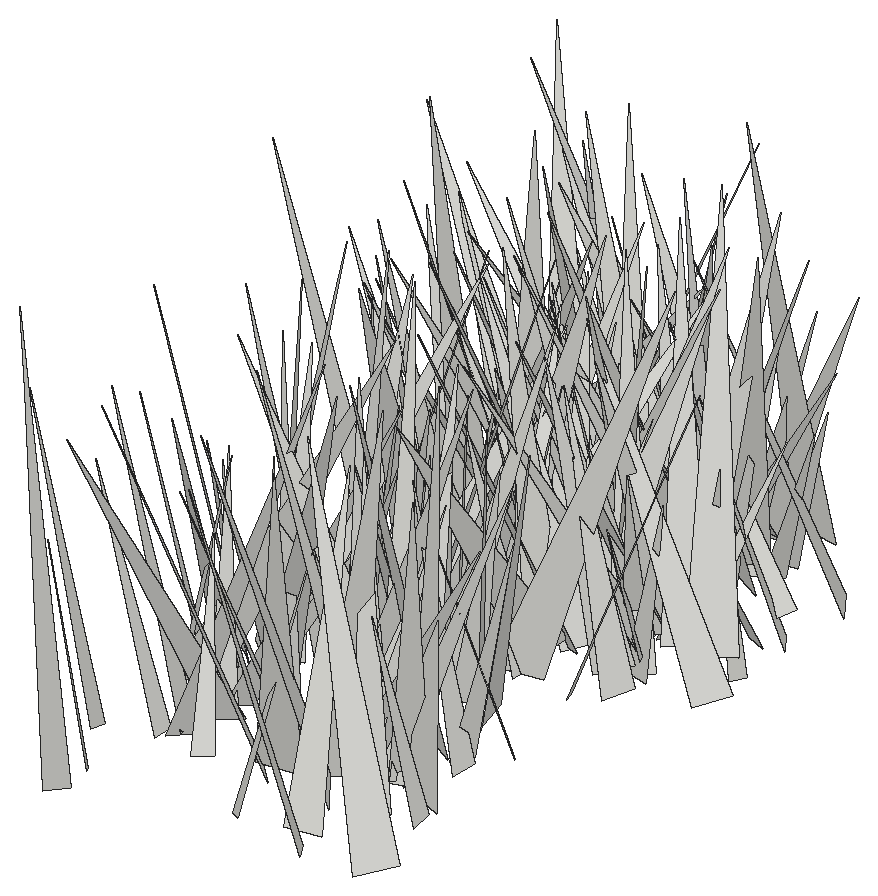
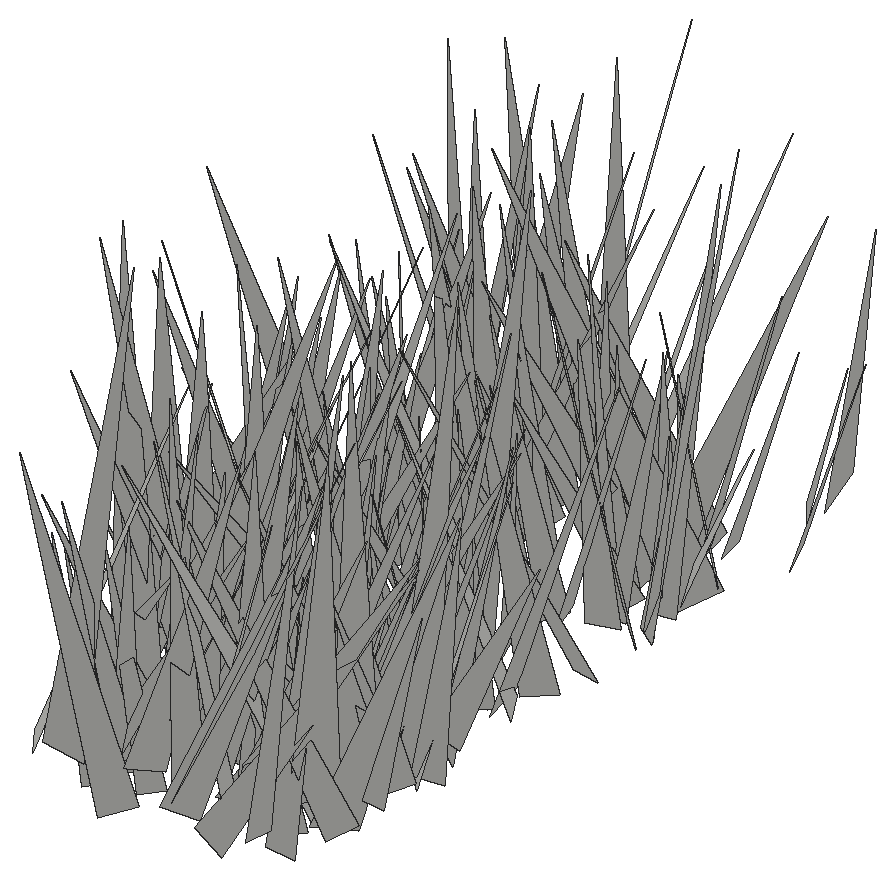
# SketchUp Ruby script. Lengths in inches.
U = 1.inch
M = Sketchup.active_model
def pt(a) = Geom::Point3d.new(a.map { |v| v * U })
def face(e, loops, mat)
  f = e.add_face(loops[0].map { |a| pt(a) })
  loops[1..].each { |l| e.add_face(l.map { |a| pt(a) }).erase! }
  f.material = f.back_material = mat if mat
  f
end
# faces: each face lists its corners as indices into pts; further lists are holes
def faces(e, pts, list, mat = nil) = list.each { |f| face(e, (f[0].is_a?(Array) ? f : [f]).map { |l| l.map { |i| pts[i] } }, mat) }
# xy, xz, yz: faces in a plane at the given z, y or x. An outline is a flat list of corners, or four numbers for a rectangle; further outlines are holes
def ring(l) = l.size == 4 ? [[l[0], l[1]], [l[2], l[1]], [l[2], l[3]], [l[0], l[3]]] : l.each_slice(2).to_a
def flat(e, list, mat, &to3) = list.each { |f| face(e, (f[0].is_a?(Array) ? f : [f]).map { |l| ring(l).map { |u, v| to3.(u, v) } }, mat) }
def xy(e, z, list, mat = nil) = flat(e, list, mat) { |x, y| [x, y, z] }
def xz(e, y, list, mat = nil) = flat(e, list, mat) { |x, z| [x, y, z] }
def yz(e, x, list, mat = nil) = flat(e, list, mat) { |y, z| [x, y, z] }
def lines(e, pts, list) = list.each { |a, b| e.add_line(pt(pts[a]), pt(pts[b])) }
# prism: a flat outline (further loops are holes) pulled along v
def prism(e, loops, v, mat = nil)
  f = face(e, loops, mat); d = Geom::Vector3d.new(v.map { |x| x * U })
  f.pushpull(f.normal.samedirection?(d) ? d.length : -d.length)
end
def box(e, o, s, mat = nil) = prism(e, [[o, [o[0] + s[0], o[1], o[2]], [o[0] + s[0], o[1] + s[1], o[2]], [o[0], o[1] + s[1], o[2]]]], [0, 0, s[2]], mat)
def at(x, y, z, deg = 0) = Geom::Transformation.translation(pt([x, y, z])) * Geom::Transformation.rotation(ORIGIN, Z_AXIS, deg.degrees)
def axes(o, x, y, z) = Geom::Transformation.new([*x, 0, *y, 0, *z, 0, *pt(o).to_a, 1])
def part(name) = M.definitions.add(name)
# library, detail: a bought-in or finely detailed component or shape, given as its bounding box
def library(name, o, s) = part(name).tap { |d| box(d.entities, o, s) }
def detail(e, o, s) = box(e.add_group.entities, o, s)
def put(e, d, t, mat = nil) = e.add_instance(d, t).tap { |i| i.material = mat if mat }
def group(e, t, mat = nil) = e.add_group.tap { |g| g.transformation = t; g.material = mat if mat }.entities
root = M.entities
c1 = part("fur_instance\#9")
p = [[0.8125,0,1.79],[0.67,-0.02,1.48],[0,-0.11,0],[0,0.11,0]]
faces(c1.entities,p,[[0,1,2,3]])
put(root,c1,axes([64.625,49.125,-27.1],[-5.41168,-1.42657,0.35166],[-1.45652,5.03228,-1.99993],[-0.1932,2.0214,5.22701]))
put(root,c1,axes([66,62.07,-27.1],[-7.51977,-1.08655,0.44758],[-1.14316,7.43533,-1.15625],[0.27218,1.20961,7.50937]))
put(root,c1,axes([65.96,65.12,-27.1],[-1.87407,5.07403,0.37598],[4.58214,1.50899,2.47512],[-2.21159,-1.17322,4.80954]))
put(root,c1,axes([65.81,53.42,-27.1],[-4.45593,-2.02584,0.38216],[-1.95722,3.87117,-2.29973],[-0.64758,2.23951,4.32095]))
put(root,c1,axes([66.16,45.11,-27.1],[-7.80069,-0.47128,0.71432],[-0.70737,7.23754,-2.94972],[0.48165,2.99651,7.23686]))
put(root,c1,axes([66.33,70.11,-28.22],[-5.80896,4.38047,0.69826],[4.41604,5.60261,1.59041],[-0.41794,-1.68592,7.09952]))
put(root,c1,axes([65.27,69.72,-27.1],[-1.60239,4.56784,1.22355],[4.62571,1.24567,1.40748],[-0.98238,-1.58525,4.63161]))
put(root,c1,axes([64.7,67.48,-27.1],[-2.06507,4.56305,1.47225],[4.79287,1.92061,0.77009],[-0.13147,-1.65628,4.94903]))
put(root,c1,axes([64.83,67.94,-27.1],[-3.71629,-3.62879,0.54604],[-3.4741,3.72939,1.13989],[1.18191,-0.44788,5.0675]))
put(root,c1,axes([66.11,46.76,-27.1],[-3.1769,-1.92196,0.83625],[-2.09296,2.82701,-1.45378],[-0.11299,1.67333,3.4166]))
put(root,c1,axes([66.51,50.08,-27.1],[-4.63616,-0.58897,0.33378],[-0.62989,4.59941,-0.63319],[0.24806,0.67142,4.63033]))
put(root,c1,axes([65.06,55.98,-27.1],[-2.14945,-3.42966,1.0737],[-3.50191,2.27993,0.27214],[0.80747,0.75821,4.03839]))
put(root,c1,axes([66.93,50.87,-27.1],[-5.59376,-1.56322,0.76508],[-1.67452,5.53596,-0.93185],[0.47433,1.10847,5.73284]))
put(root,c1,axes([65.12,56.01,-27.1],[-4.90749,-6.3294,1.61985],[-6.13533,5.16095,1.5783],[2.24565,0.26836,7.85199]))
put(root,c1,axes([66.7,70.65,-27.1],[-6.24341,4.5177,1.05822],[4.50521,6.32678,-0.4296],[1.11019,-0.26807,7.69449]))
put(root,c1,axes([66.59,64.2,-28.22],[-3.28868,-4.79968,1.75844],[-5.10998,3.14053,-0.98472],[0.13097,2.01112,5.73434]))
put(root,c1,axes([65.47,67.25,-27.1],[-0.06707,-7.91469,2.47451],[-8.29222,0.04381,-0.08466],[-0.06773,2.47503,7.91452]))
put(root,c1,axes([66.27,54.17,-27.1],[1.10778,3.32388,1.25845],[3.28018,-1.46364,0.97838],[-1.36832,-0.8177,3.36424]))
put(root,c1,axes([67.79,56.82,-27.1],[-6.22819,-1.34042,0.61243],[-1.44458,6.07908,-1.38568],[0.29149,1.48668,6.21828]))
put(root,c1,axes([66.37,66.87,-27.1],[-5.34659,-1.99732,0.9572],[-1.60106,5.21354,1.93576],[1.5304,-1.52357,5.36919]))
put(root,c1,axes([68.33,66.69,-27.1],[-4.54723,-4.75664,0.92618],[-4.80738,4.26788,-1.68375],[-0.61038,1.82216,6.36144]))
put(root,c1,axes([69.69,70.75,-28.22],[-5.05806,4.73106,0.08976],[4.36112,4.60989,2.7757],[-1.83619,-2.08349,6.34527]))
put(root,c1,axes([65.49,67.88,-27.1],[3.79033,1.52401,0.8214],[1.29616,-3.80865,1.0854],[-1.14773,0.73179,3.93842]))
put(root,c1,axes([65.54,56.25,-27.1],[4.64173,5.41011,1.53464],[5.42173,-4.8336,0.64123],[-1.49305,-0.73288,7.09956]))
put(root,c1,axes([65.36,61.04,-27.1],[2.82826,-4.43632,2.67471],[-5.15951,-2.68482,1.00262],[-0.46309,2.81866,5.16476]))
put(root,c1,axes([68.84,73.27,-28.22],[-0.73144,-5.99959,0.26703],[-5.39662,0.53861,-2.681],[-2.63493,0.56233,5.41685]))
put(root,c1,axes([67.57,52.08,-27.1],[0.6668,-6.36542,0.43774],[-6.10772,-0.7641,-1.80742],[-1.84553,0.22889,6.13974]))
put(root,c1,axes([66.61,73.57,-27.1],[-5.67591,-0.59927,2.29984],[-0.30227,6.08824,0.84044],[2.35734,-0.66225,5.64524]))
put(root,c1,axes([65.61,51.87,-27.1],[3.51843,3.11531,1.14482],[3.25687,-3.56198,-0.31656],[-0.63919,-1.00114,4.68874]))
put(root,c1,axes([65.48,62.2,-27.1],[5.06961,3.19969,0.78256],[3.08145,-5.11429,0.94868],[-1.16407,0.39664,5.91937]))
put(root,c1,axes([66.59,56.34,-27.1],[-1.35199,5.16754,1.66066],[5.39955,1.4549,-0.13134],[0.55327,-1.57128,5.33986]))
put(root,c1,axes([67.92,59.5625,-27.1],[-5.24858,-0.93793,1.2858],[-1.33069,5.01688,-1.77222],[0.87308,2.00792,5.02857]))
put(root,c1,axes([65.54,54.71,-27.1],[-1.80775,-6.68688,0.47497],[-6.40102,1.86794,1.93536],[1.9917,-0.06601,6.65106]))
put(root,c1,axes([67.4,68.64,-27.1],[-5.6995,-3.45113,0.56108],[-3.05969,5.44221,2.39374],[1.69215,-1.78365,6.21808]))
put(root,c1,axes([67.09,52.47,-27.1],[-1.17354,4.22506,1.16991],[4.38332,1.15287,0.2334],[0.0799,-1.19029,4.3788]))
put(root,c1,axes([68.92,65.9,-27.1],[-2.19806,-5.17129,0.07017],[-4.98418,2.09779,-1.52836],[-1.38027,0.66005,5.4072]))
put(root,c1,axes([66.33,69.02,-27.1],[-4.86484,4.13925,3.64162],[4.78109,5.5858,0.03796],[2.74517,-2.39309,6.38738]))
put(root,c1,axes([68.05,63.3,-27.1],[-6.59248,-1.12335,1.64682],[-1.04061,6.79216,0.46743],[1.70031,-0.1986,6.67115]))
put(root,c1,axes([66.55,55.8,-27.1],[-0.44013,-4.40012,0.04518],[-4.35564,0.44209,0.62427],[0.62566,-0.01764,4.37779]))
put(root,c1,axes([65.02,59.18,-27.1],[2.4491,6.4359,0.09226],[6.32974,-2.3903,-1.28384],[1.16776,-0.54137,6.7654]))
put(root,c1,axes([70.14,73.03,-27.1],[-7.66892,-1.90839,0.15613],[-1.91216,7.66661,-0.21311],[0.09999,0.24454,7.89993]))
put(root,c1,axes([68.79,66.84,-28.22],[-4.89818,0.93846,0.55806],[1.01529,4.8584,0.74127],[0.40164,-0.83642,4.93188]))
put(root,c1,axes([67.65,54.57,-27.1],[-6.13991,-1.94187,2.86824],[-2.65031,6.39227,-1.34568],[2.23013,2.25037,6.2975]))
put(root,c1,axes([66.64,72.42,-28.22],[-2.27672,-7.40144,1.23154],[-7.29478,2.48469,1.44709],[1.75622,0.72557,7.60728]))
put(root,c1,axes([68.75,71.23,-27.1],[0.69444,-4.60057,1.02449],[-4.36557,-1.0182,-1.61314],[-1.77671,0.70364,4.36409]))
put(root,c1,axes([69.07,68.81,-28.22],[-2.8111,-5.64649,0.53318],[-5.64839,2.7334,-0.83291],[-0.51273,0.84565,6.25232]))
put(root,c1,axes([65.1,68.59,-27.1],[5.86888,-2.59714,0.14419],[-2.59865,-5.83866,0.60558],[0.11385,0.61201,6.38922]))
put(root,c1,axes([67.4,64.04,-27.1],[3.19373,2.97376,0.94617],[2.91746,-3.32577,0.60507],[-1.10768,-0.18543,4.3217]))
put(root,c1,axes([66.19,62.79,-27.1],[-0.42992,-4.68733,0.89248],[-4.33891,0.75688,1.88505],[1.98531,0.63912,4.31306]))
put(root,c1,axes([68.4375,49.73,-27.1],[-2.65941,2.49787,0.36396],[2.46932,2.68404,-0.37765],[0.52369,0.0288,3.62894]))
put(root,c1,axes([69.45,73.93,-27.1],[3.15853,-4.87453,2.05329],[-4.28659,-3.76007,-2.33247],[-3.09874,0.23284,5.31949]))
put(root,c1,axes([70.11,71.71,-27.1],[-5.34119,3.3335,0.99515],[3.47843,5.14626,1.43085],[0.05516,-1.74201,6.13133]))
put(root,c1,axes([67.03,50.33,-27.1],[6.5419,0.41912,1.71437],[-0.23349,-6.31856,2.43568],[-1.74935,2.41069,6.08602]))
put(root,c1,axes([66.8125,63.14,-27.1],[7.11754,-4.23376,0.53848],[-3.90576,-6.88369,-2.49681],[-1.7204,-1.88792,7.89621]))
put(root,c1,axes([67.07,71.17,-28.22],[1.8239,-3.22944,0.77362],[-3.28665,-1.6292,0.94764],[0.47508,1.1273,3.58579]))
put(root,c1,axes([70.16,70.29,-27.1],[-2.19401,4.08598,0.64459],[3.98986,1.89782,1.55038],[-1.09165,-1.27572,4.37096]))
put(root,c1,axes([64.6875,71.76,-27.1],[2.58062,-5.27777,0.62862],[-4.46822,-1.77579,3.43383],[2.87837,1.97518,4.76689]))
put(root,c1,axes([70.27,51.87,-27.1],[-6.71472,0.14595,1.05093],[-0.21339,6.41005,-2.25365],[1.03933,2.25902,6.32691]))
put(root,c1,axes([69.97,64.77,-28.22],[-3.16034,-1.96863,0.75138],[-2.10046,2.8354,-1.40585],[-0.16774,1.5852,3.44773]))
put(root,c1,axes([67.62,66.48,-28.22],[1.29367,6.30142,0.29631],[6.29029,-1.26564,-0.54746],[0.47747,-0.39942,6.4095]))
put(root,c1,axes([69.52,73.01,-27.1],[-3.89073,-3.2521,0.98713],[-3.3181,3.95947,-0.03367],[0.73538,0.65937,5.07078]))
put(root,c1,axes([70.61,50.16,-27.1],[-5.16383,-5.19186,0.43743],[-5.2089,5.15828,-0.26709],[0.11856,0.49863,7.31773]))
put(root,c1,axes([69.6,51.85,-27.1],[-4.54245,-0.30979,1.16713],[-0.64985,4.4561,-1.34644],[1.01777,1.46262,4.34936]))
put(root,c1,axes([69.37,52.73,-27.1],[-3.58338,-3.97137,0.418],[-3.89573,3.60001,0.80641],[0.87736,-0.23507,5.28792]))
put(root,c1,axes([67.5625,65.23,-28.22],[3.70802,-0.97097,0.29213],[-0.94384,-3.70994,-0.3508],[-0.37053,-0.26665,3.81695]))
put(root,c1,axes([70.13,70.26,-27.1],[-6.35948,3.06032,1.72749],[3.24757,6.48259,0.47123],[1.34279,-1.18457,7.04176]))
put(root,c1,axes([65.21,53.34,-27.1],[6.5519,-4.81181,0.9912],[-4.80718,-5.93833,2.94799],[1.01342,2.94042,7.57563]))
put(root,c1,axes([67.26,62.46,-27.1],[0.04423,5.29855,0.55334],[5.02486,0.14232,-1.76445],[1.76963,-0.53655,4.99632]))
put(root,c1,axes([70.47,69.22,-27.1],[-6.55915,2.85076,0.80174],[2.70921,6.56329,-1.17278],[1.19574,0.76707,7.05506]))
put(root,c1,axes([66.72,54.75,-27.1],[3.29977,-2.51906,0.3221],[-2.3698,-2.86445,1.87534],[0.91296,1.66948,3.70368]))
put(root,c1,axes([68.71,61.32,-27.1],[3.22144,-2.0672,0.86258],[-1.86043,-3.31076,-0.98626],[-1.24746,-0.40075,3.69841]))
put(root,c1,axes([68.41,67.81,-28.22],[1.07751,-3.9043,2.33703],[-4.53898,-0.75293,0.83488],[0.32078,2.46086,3.96327]))
put(root,c1,axes([69.34,56.67,-27.1],[-4.14484,-0.82966,2.07391],[-1.4546,4.32013,-1.17886],[1.69516,1.67847,4.05935]))
put(root,c1,axes([67.32,53.02,-27.1],[6.04009,-0.71684,0.90558],[-1.00409,-5.64184,2.23115],[-0.57074,2.3393,5.65849]))
put(root,c1,axes([67.7,69.1875,-28.22],[6.85876,3.23862,0.41321],[3.02392,-6.66397,2.03701],[-1.23097,1.67477,7.30628]))
put(root,c1,axes([69.11,71.08,-27.1],[3.4639,-0.21189,1.20284],[0.06017,-3.58323,-0.80448],[-1.21988,-0.7784,3.37584]))
put(root,c1,axes([70.94,63.43,-27.1],[2.36274,4.29484,1.97791],[3.91667,-3.01643,1.87116],[-2.64906,-0.62918,4.53067]))
put(root,c1,axes([71.33,67.07,-28.22],[-4.99004,2.24313,0.58277],[2.2784,5.00139,0.2583],[0.42444,-0.4756,5.46492]))
put(root,c1,axes([69.54,61.42,-27.1],[3.09242,2.58599,1.68004],[2.84079,-3.31463,-0.12697],[-1.19992,-1.18273,4.02918]))
put(root,c1,axes([70.6,67.11,-28.22],[-3.32365,-1.7064,1.24939],[-2.04417,3.18881,-1.08271],[0.54234,1.56176,3.57578]))
put(root,c1,axes([72.54,54.74,-27.1],[-7.38136,0.22251,0.33251],[0.26326,7.32737,0.9407],[0.30128,-0.95116,7.32455]))
put(root,c1,axes([68.13,56.85,-27.1],[4.67852,-1.7119,0.20248],[-1.71617,-4.68064,0.08066],[-0.16239,0.14538,4.98123]))
put(root,c1,axes([69.04,66.99,-28.22],[4.65411,-4.15615,0.09318],[-4.0063,-4.52139,-1.56511],[-1.10988,-1.10744,6.04026]))
put(root,c1,axes([67.3,54.8,-27.1],[7.07591,-3.11018,0.05148],[-3.09924,-7.06002,-0.5432],[-0.26559,-0.47663,7.71016]))
put(root,c1,axes([68.98,63.45,-27.1],[3.85375,-0.57416,0.66525],[-0.65849,-3.86826,0.47595],[-0.58191,0.57487,3.8671]))
put(root,c1,axes([68.12,65.98,-28.22],[-0.23722,4.19444,0.05409],[3.55446,0.22976,-2.22834],[2.22756,0.08005,3.56147]))
put(root,c1,axes([72.9,66.01,-28.22],[-7.48937,-0.81173,0.36322],[-0.84224,7.4632,-0.68756],[0.28542,0.72333,7.50179]))
put(root,c1,axes([68.73,72.05,-28.22],[6.14666,2.4589,1.36982],[2.59506,-6.2248,-0.47069],[-1.09008,-0.95377,6.60349]))
put(root,c1,axes([71.31,53.25,-27.1],[2.8075,7.47142,1.47372],[7.21104,-3.11318,2.04573],[-2.44844,-0.60171,7.71486]))
put(root,c1,axes([70.05,64.76,-27.1],[-2.01295,-3.23513,0.63988],[-3.06607,2.112,1.03257],[1.21439,-0.03018,3.66768]))
put(root,c1,axes([72.03,72.48,-27.1],[-5.02266,3.34128,1.54054],[3.64584,4.87057,1.32283],[0.49523,-1.96924,5.88569]))
put(root,c1,axes([71.11,65.16,-28.22],[-4.06626,4.25963,1.22614],[4.27905,4.20638,-0.4224],[1.15655,-0.5867,5.87371]))
put(root,c1,axes([71.48,64.51,-27.1],[-3.55756,1.9012,0.49829],[1.88183,3.59228,-0.2708],[0.56709,0.00632,4.02461]))
put(root,c1,axes([71.13,61.78,-27.1],[-3.68775,-0.43694,1.2324],[0.03671,3.65173,1.40455],[1.30705,-1.33536,3.43768]))
put(root,c1,axes([73.31,62.43,-27.1],[-3.41079,-4.86692,0.40111],[-4.72199,3.16213,-1.78467],[-1.24525,1.33989,5.66881]))
put(root,c1,axes([68.41,64.77,-28.22],[0.11593,7.32982,3.76994],[7.80213,1.11829,-2.4142],[2.6581,-3.60212,6.9218]))
put(root,c1,axes([72.18,69.73,-28.22],[2.04194,-5.37013,1.21962],[-4.97283,-2.35693,-2.05211],[-2.36574,0.31918,5.36625]))
put(root,c1,axes([71.54,65.4,-27.1],[-3.81436,-7.20009,0.2192],[-7.12697,3.80817,1.069],[1.0467,-0.30859,8.07762]))
put(root,c1,axes([68.99,63.5,-28.22],[-1.44675,6.62808,0.1342],[5.91861,1.35324,-3.03008],[2.98656,0.529,6.06986]))
put(root,c1,axes([69.64,64.05,-27.1],[4.05743,2.55482,1.17911],[2.80714,-3.81746,-1.3882],[-0.19333,-1.81108,4.58942]))
put(root,c1,axes([71.45,62.89,-27.1],[2.88206,-3.90926,2.29022],[-4.22914,-3.29495,-0.30223],[-1.62535,1.64154,4.8474]))
put(root,c1,axes([71.9375,61.28,-27.1],[-3.2921,4.67046,0.35788],[4.62081,3.30978,-0.68745],[0.76768,0.10645,5.67261]))
put(root,c1,axes([74.22,64.76,-28.22],[-6.31151,-2.93767,0.11387],[-2.9284,6.25835,-0.85765],[-0.25951,0.82534,6.90866]))
put(root,c1,axes([73.45,62.86,-27.1],[-4.72001,4.32069,1.36462],[4.52973,4.45158,1.57294],[-0.11027,-2.07946,6.20264]))
put(root,c1,axes([69.66,73.18,-27.1],[6.23542,-1.61716,0.46655],[-1.48447,-6.12774,-1.40019],[-0.79324,-1.24458,6.2877]))
put(root,c1,axes([71.67,47.33,-27.1],[2.88186,3.44939,0.31018],[3.15851,-2.7832,1.60537],[-1.42067,0.8094,4.19835]))
put(root,c1,axes([72.45,62.29,-27.1],[-6.37075,2.32719,2.17346],[2.54476,6.64308,0.34616],[1.91413,-1.08621,6.77365]))
put(root,c1,axes([72.74,68.92,-28.22],[-1.86081,5.49202,1.44787],[5.66351,1.67938,0.90859],[-0.42807,-1.65488,5.72707]))
put(root,c1,axes([70.37,57.85,-27.1],[6.70956,3.50603,1.11128],[3.28027,-6.75003,1.49074],[-1.66343,0.8308,7.42214]))
put(root,c1,axes([73.56,72.32,-27.1],[-2.21504,-4.22644,0.02495],[-4.06696,2.12371,-1.31133],[-1.15036,0.62998,4.58799]))
put(root,c1,axes([72.3125,69.38,-27.1],[-4.28655,1.17606,1.86698],[1.8295,4.17484,1.57066],[1.23356,-2.10497,4.15821]))
put(root,c1,axes([73.9375,51.52,-27.1],[-6.93543,-2.32629,0.88421],[-2.41004,6.93097,-0.66862],[0.62063,0.91853,7.28456]))
put(root,c1,axes([71.12,57.4,-27.1],[-1.84691,-6.18778,0.26193],[-5.9057,1.84189,1.87043],[1.86547,-0.29517,6.18071]))
put(root,c1,axes([73.79,69.28,-28.22],[-6.95078,-0.2098,1.40903],[-0.48679,6.94525,-1.36721],[1.33881,1.43604,6.81821]))
put(root,c1,axes([70.57,58.61,-27.1],[4.90607,-3.46037,0.24315],[-3.44997,-4.91123,-0.28332],[-0.36191,-0.09172,5.99695]))
put(root,c1,axes([74.77,46.83,-27.1],[-5.23852,-3.39609,0.6769],[-3.443,4.97658,-1.67721],[-0.37061,1.77027,6.01352]))
put(root,c1,axes([70.88,50.57,-27.1],[2.24537,-6.9608,0.71668],[-6.96969,-2.1575,0.8813],[0.62434,0.94895,7.26069]))
put(root,c1,axes([73.04,60.47,-27.1],[-4.43499,0.78648,1.49873],[1.10021,4.53377,0.87655],[1.28619,-1.16631,4.41807]))
put(root,c1,axes([74.96,67.24,-28.22],[-6.90561,-3.33755,0.10935],[-3.32242,6.89219,0.54573],[0.33571,-0.44394,7.65042]))
put(root,c1,axes([73.01,50.48,-27.1],[-6.10663,-5.12788,1.30944],[-4.81653,6.21333,1.86984],[2.19336,-0.63253,7.75176]))
put(root,c1,axes([74.29,52.1,-27.1],[0.27633,8.1596,0.76138],[7.93766,-0.45592,2.00518],[-2.0377,-0.66947,7.91421]))
put(root,c1,axes([72.625,52.87,-27.1],[-4.98307,4.13485,3.06586],[4.6284,5.46651,0.15019],[2.25263,-2.08511,6.47344]))
put(root,c1,axes([72.41,67.45,-27.1],[-0.34138,-6.1128,0.75859],[-6.1403,0.39794,0.44341],[0.48829,0.7305,6.10625]))
put(root,c1,axes([71.3,58.45,-27.1],[2.20928,6.37096,1.50715],[6.50914,-1.9672,-1.22586],[0.70121,-1.81177,6.63078]))
put(root,c1,axes([74.41,67.76,-27.1],[-0.98604,-7.77609,1.14314],[-7.75331,0.77346,-1.42635],[-1.28859,1.29646,7.70749]))
put(root,c1,axes([75.43,63.38,-27.1],[-5.24793,-3.08562,0.82091],[-3.15493,4.76816,-2.24651],[-0.49124,2.34081,5.65818]))
put(root,c1,axes([72.81,61.85,-27.1],[6.08431,-4.17162,0.61258],[-3.3903,-5.47976,-3.64343],[-2.50671,-2.71408,6.41457]))
put(root,c1,axes([72.18,64.79,-27.1],[1.68223,-3.64936,0.16027],[-3.63941,-1.65928,0.41825],[0.31341,0.31999,3.9966]))
put(root,c1,axes([73.68,71.39,-28.22],[2.76185,-3.07557,2.49035],[-3.57907,-3.23702,-0.02845],[-1.68858,1.83068,4.13354]))
put(root,c1,axes([72.21,71.88,-28.22],[2.46707,-3.42013,1.11602],[-3.59628,-2.30764,0.87798],[0.09798,1.4166,4.12467]))
put(root,c1,axes([73.02,66.79,-28.22],[-1.28259,-7.19659,1.19017],[-7.23451,1.40948,0.72639],[0.93233,1.03678,7.27381]))
put(root,c1,axes([73.53,54.05,-27.1],[-4.06355,5.05875,1.67662],[5.05755,4.32523,-0.79246],[1.68023,-0.78477,6.44014]))
put(root,c1,axes([71.875,52.65,-27.1],[6.69974,-1.69034,1.74311],[-2.11177,-6.58131,1.73465],[-1.19837,2.1474,6.68841]))
put(root,c1,axes([73.54,68.26,-28.22],[1.95949,2.80373,1.45551],[3.04239,-2.136,0.01872],[-0.85045,-1.18135,3.42055]))
put(root,c1,axes([74.39,65.32,-27.1],[-1.51656,-6.50321,0.08888],[-6.50028,1.51258,-0.24097],[-0.21452,0.14123,6.67335]))
put(root,c1,axes([74.58,64.46,-27.1],[-5.86145,-3.99032,0.23805],[-3.68658,5.55942,2.41617],[1.54546,-1.87245,6.66644]))
put(root,c1,axes([74.02,47.84,-27.1],[-1.14776,6.0133,0.84328],[6.0716,1.14805,0.07727],[0.08148,-0.84289,6.12137]))
put(root,c1,axes([73.88,54.87,-27.1],[-3.21608,-6.87634,1.40534],[-6.91778,3.36666,0.64196],[1.18463,0.99184,7.56406]))
put(root,c1,axes([74.45,52.43,-27.1],[-5.1152,1.11044,1.16629],[0.73583,5.06638,-1.59654],[1.43244,1.36283,4.98492]))
put(root,c1,axes([74.63,63.87,-28.22],[-5.4488,4.52209,1.619],[4.59694,5.6194,-0.22458],[1.39234,-0.85616,7.07731]))
put(root,c1,axes([72.83,57.7,-27.1],[2.7967,-3.72992,1.22325],[-3.91864,-2.74089,0.60164],[-0.23004,1.34365,4.62297]))
put(root,c1,axes([70.46,65.98,-27.1],[6.41393,4.45568,0.74677],[4.39818,-5.86174,-2.80093],[1.0328,-2.70854,7.29015]))
put(root,c1,axes([73.29,64.82,-27.1],[6.28919,2.00514,2.27548],[2.25266,-6.59596,-0.4138],[-2.03074,-1.10685,6.58812]))
put(root,c1,axes([74.52,64.59,-27.1],[0.87067,-3.63818,0.96208],[-3.64876,-1.05785,-0.69825],[-0.92116,0.75142,3.67517]))
put(root,c1,axes([72.9,72.21,-27.1],[4.30722,-1.10997,0.82887],[-1.21703,-4.32511,0.53238],[-0.66174,0.72977,4.41597]))
put(root,c1,axes([73.49,51.28,-27.1],[1.79121,4.66243,0.42191],[4.67903,-1.79759,0.00003],[-0.15134,-0.39383,4.99466]))
put(root,c1,axes([72.62,51.36,-27.1],[5.72788,-5.11466,1.67521],[-5.30647,-5.77538,0.51083],[-0.89854,1.50329,7.66207]))
put(root,c1,axes([74.9375,50.18,-27.1],[1.5886,-5.12639,3.23902],[-5.9044,-2.07062,-0.3813],[-1.38174,2.95423,5.35333]))
put(root,c1,axes([74.39,56.42,-27.1],[4.38059,2.58911,2.20412],[2.75267,-4.81057,0.18002],[-1.99611,-0.9519,5.08534]))
put(root,c1,axes([75.55,54.1875,-27.1],[-4.97388,0.03891,0.99351],[0.0174,5.07103,-0.11152],[0.99411,0.10595,4.97278]))
put(root,c1,axes([74.72,73.1875,-27.1],[-1.19832,-8.06423,2.00487],[-8.30399,1.23724,0.01324],[0.30817,1.98109,8.15276]))
put(root,c1,axes([72.24,73.52,-28.22],[4.49175,-3.99144,0.42922],[-3.97143,-4.32409,1.3497],[0.58618,1.28931,5.8554]))
put(root,c1,axes([72.91,63.86,-27.1],[-0.40245,7.17423,1.83924],[7.10701,0.89237,-1.92572],[2.08393,-1.65784,6.92265]))
put(root,c1,axes([75.2,62.26,-27.1],[3.86572,-4.28586,2.24353],[-4.19582,-4.39988,-1.17556],[-2.40771,0.7863,5.6507]))
put(root,c1,axes([75.15,69.17,-27.1],[-2.33347,-4.94017,0.88075],[-4.99474,2.38012,0.11709],[0.48332,0.74554,5.4623]))
put(root,c1,axes([76.41,68.02,-28.22],[-2.68226,-4.58353,0.12394],[-4.53778,2.63294,-0.83358],[-0.65781,0.52677,5.24485]))
put(root,c1,axes([73.99,64.97,-28.22],[3.06057,-3.28635,0.3748],[-3.27189,-3.08287,-0.31361],[-0.4851,0.05914,4.47983]))
put(root,c1,axes([76.02,64.92,-27.1],[-5.00326,5.02156,1.24961],[5.08502,5.09325,-0.10752],[0.95924,-0.80806,7.08781]))
put(root,c1,axes([75.18,65.36,-27.1],[2.93992,-5.13493,1.13143],[-5.01799,-3.12719,-1.15379],[-1.5708,0.37938,5.8034]))
put(root,c1,axes([77.21,68.5625,-27.1],[-1.66623,3.3763,0.05798],[2.90925,1.40249,1.93607],[-1.71436,-0.9015,3.22914]))
put(root,c1,axes([73.99,57.53,-27.1],[5.32416,0.8497,1.29821],[1.01973,-5.41351,-0.63884],[-1.1694,-0.85204,5.35356]))
put(root,c1,axes([73.15,70.35,-27.1],[4.12414,-1.44643,0.07491],[-1.4095,-3.95608,1.21201],[0.33327,1.1677,4.19901]))
put(root,c1,axes([76.33,61.1,-27.1],[-4.97411,1.9133,1.24146],[2.05101,5.05519,0.42681],[0.99764,-0.85328,5.31228]))
put(root,c1,axes([73.93,66.6875,-28.22],[6.79493,0.95964,1.40947],[0.56386,-6.72962,1.86359],[-1.60922,1.6941,6.60447]))
put(root,c1,axes([77.15,71.64,-28.22],[-5.5722,-4.07145,0.43281],[-4.071,5.58734,0.1482],[0.43699,0.13539,6.89957]))
put(root,c1,axes([74.61,68.4,-28.22],[4.01633,-1.15722,1.23996],[-1.33038,-4.12648,0.45808],[-1.05202,0.80037,4.15454]))
put(root,c1,axes([77.45,47.32,-27.1],[-6.20404,3.776,0.73856],[3.82283,6.20814,0.37243],[0.43544,-0.70326,7.25325]))
put(root,c1,axes([73.9,72.58,-28.22],[2.06201,-3.51619,0.27094],[-3.44771,-1.94389,1.0117],[0.74186,0.73932,3.94867]))
put(root,c1,axes([72.91,60.21,-27.1],[5.54256,-5.39998,2.31392],[-5.86744,-4.92827,2.55329],[0.29519,3.43313,7.30483]))
put(root,c1,axes([74.26,71.63,-28.22],[3.14021,-1.95272,0.11029],[-1.95573,-3.13292,0.21476],[0.01996,0.24059,3.6916]))
put(root,c1,axes([72.81,52.14,-27.1],[4.53332,-3.78068,0.06575],[-3.6354,-4.32956,1.69931],[1.04008,1.34544,5.65304]))
put(root,c1,axes([75.82,56.23,-27.1],[-3.10311,-4.08719,0.56583],[-3.96021,3.14894,1.02739],[1.15846,-0.18348,5.02781]))
put(root,c1,axes([74.7,52.43,-27.1],[2.07468,-5.92746,1.15005],[-6.03286,-1.98482,0.6533],[0.24901,1.299,6.24598]))
put(root,c1,axes([78.93,62.62,-27.1],[-3.29072,5.65648,0.59206],[5.32719,2.82602,2.60955],[-1.99181,-1.7869,6.00123]))
put(root,c1,axes([74.78,63.89,-28.22],[0.44262,-3.83329,1.02735],[-3.85493,-0.16968,1.02773],[0.94293,1.1057,3.71938]))
put(root,c1,axes([74.8,67.22,-28.22],[1.90373,-3.64825,0.45227],[-3.65968,-1.83258,0.622],[0.34793,0.68584,4.0678]))
put(root,c1,axes([77.45,65.8,-28.22],[-4.50739,-0.00087,0.31518],[-0.09503,4.31184,-1.34718],[0.30051,1.35052,4.30136]))
put(root,c1,axes([75.16,60.05,-27.1],[4.59925,2.87418,0.36346],[2.61006,-4.40682,1.82035],[-1.25721,1.36572,5.10885]))
put(root,c1,axes([75.07,54.69,-27.1],[3.97041,-1.42005,1.05601],[-1.57618,-4.01704,0.5243],[-0.80459,0.86179,4.18399]))
put(root,c1,axes([76.58,50.71,-27.1],[-3.79793,-0.43925,1.06155],[-0.29859,3.91782,0.55288],[1.10936,-0.44932,3.78306]))
put(root,c1,axes([74.53,66.74,-27.1],[-0.74897,7.24815,2.93985],[7.55595,1.43371,-1.60981],[2.0214,-2.6736,7.1067]))
put(root,c1,axes([74.97,66.29,-28.22],[1.23248,3.89294,0.26564],[3.83774,-1.15903,-0.82034],[0.70519,-0.49622,4.00013]))
put(root,c1,axes([77.11,64.85,-27.1],[-4.81371,6.17541,1.55135],[6.27572,4.93015,-0.15223],[1.07597,-1.1279,7.82843]))
put(root,c1,axes([75.76,51.79,-27.1],[-2.07525,-6.86081,3.30693],[-7.48887,2.46229,0.40886],[1.38687,3.02978,7.15613]))
put(root,c1,axes([74.13,70.22,-27.1],[5.44226,-5.9088,0.26751],[-5.91243,-5.44486,0.01623],[-0.16928,0.20777,8.03317]))
put(root,c1,axes([73.9375,52.73,-27.1],[3.63408,5.21962,1.38175],[5.32326,-3.18476,-1.96987],[0.90365,-2.23003,6.04736]))
put(root,c1,axes([77.15,68.58,-28.22],[-3.54687,-2.63553,0.56126],[-2.61948,3.58991,0.30355],[0.63194,0.08835,4.40842]))
